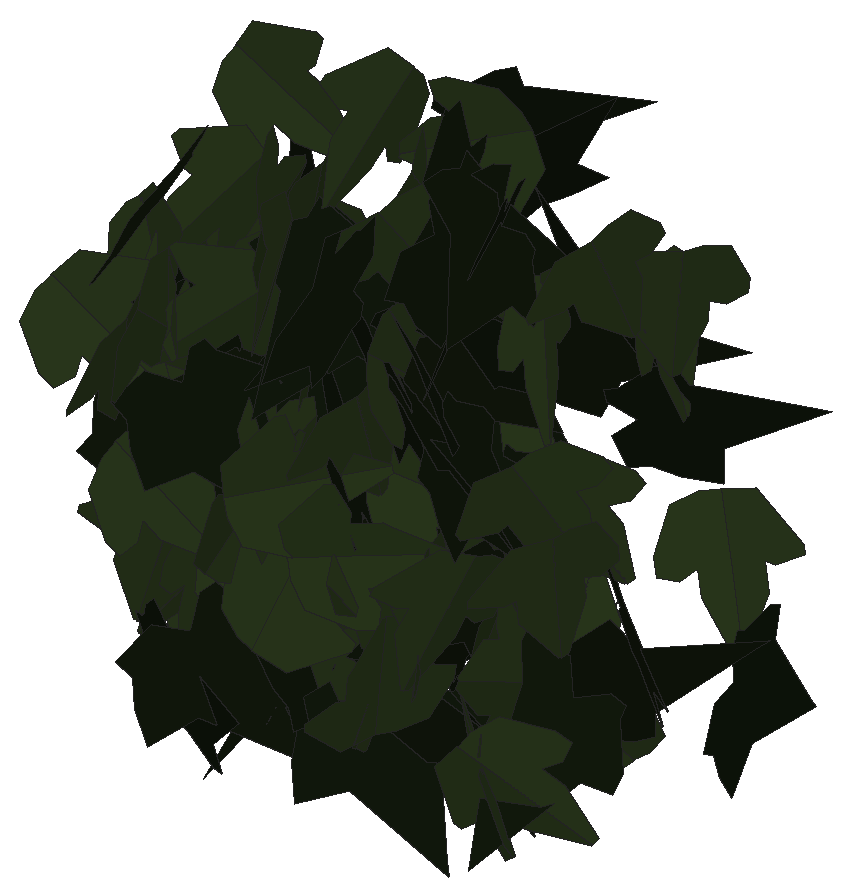
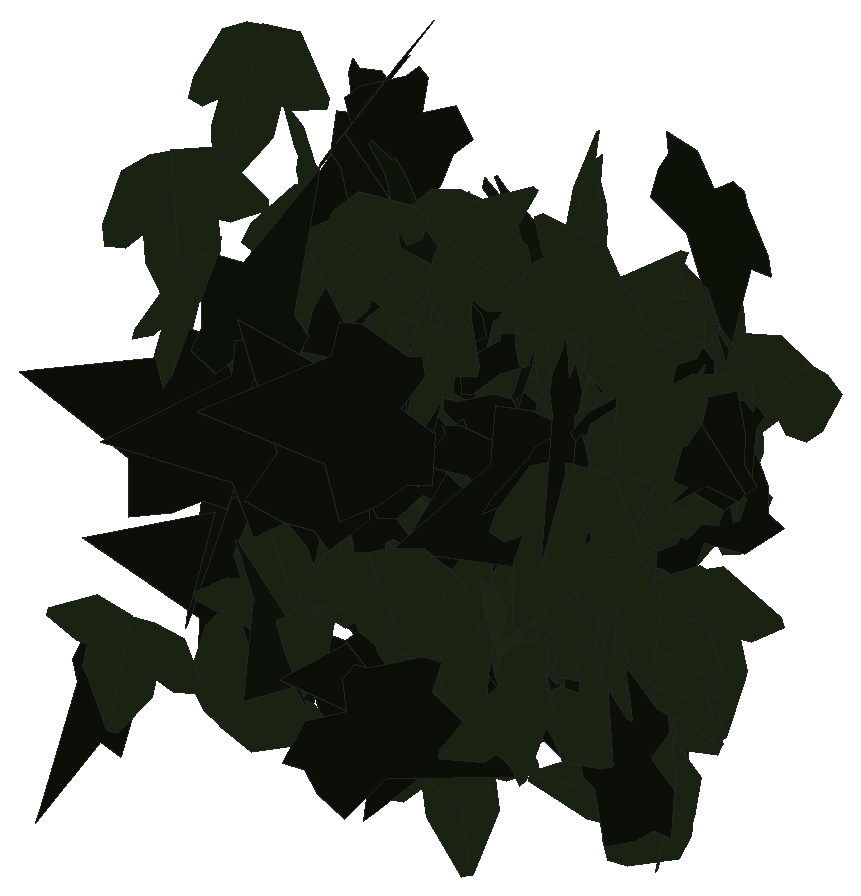
# SketchUp Ruby script. Lengths in inches.
U = 1.inch
M = Sketchup.active_model
def pt(a) = Geom::Point3d.new(a.map { |v| v * U })
def face(e, loops, mat)
  f = e.add_face(loops[0].map { |a| pt(a) })
  loops[1..].each { |l| e.add_face(l.map { |a| pt(a) }).erase! }
  f.material = f.back_material = mat if mat
  f
end
# faces: each face lists its corners as indices into pts; further lists are holes
def faces(e, pts, list, mat = nil) = list.each { |f| face(e, (f[0].is_a?(Array) ? f : [f]).map { |l| l.map { |i| pts[i] } }, mat) }
# xy, xz, yz: faces in a plane at the given z, y or x. An outline is a flat list of corners, or four numbers for a rectangle; further outlines are holes
def ring(l) = l.size == 4 ? [[l[0], l[1]], [l[2], l[1]], [l[2], l[3]], [l[0], l[3]]] : l.each_slice(2).to_a
def flat(e, list, mat, &to3) = list.each { |f| face(e, (f[0].is_a?(Array) ? f : [f]).map { |l| ring(l).map { |u, v| to3.(u, v) } }, mat) }
def xy(e, z, list, mat = nil) = flat(e, list, mat) { |x, y| [x, y, z] }
def xz(e, y, list, mat = nil) = flat(e, list, mat) { |x, z| [x, y, z] }
def yz(e, x, list, mat = nil) = flat(e, list, mat) { |y, z| [x, y, z] }
def lines(e, pts, list) = list.each { |a, b| e.add_line(pt(pts[a]), pt(pts[b])) }
# prism: a flat outline (further loops are holes) pulled along v
def prism(e, loops, v, mat = nil)
  f = face(e, loops, mat); d = Geom::Vector3d.new(v.map { |x| x * U })
  f.pushpull(f.normal.samedirection?(d) ? d.length : -d.length)
end
def box(e, o, s, mat = nil) = prism(e, [[o, [o[0] + s[0], o[1], o[2]], [o[0] + s[0], o[1] + s[1], o[2]], [o[0], o[1] + s[1], o[2]]]], [0, 0, s[2]], mat)
def at(x, y, z, deg = 0) = Geom::Transformation.translation(pt([x, y, z])) * Geom::Transformation.rotation(ORIGIN, Z_AXIS, deg.degrees)
def axes(o, x, y, z) = Geom::Transformation.new([*x, 0, *y, 0, *z, 0, *pt(o).to_a, 1])
def part(name) = M.definitions.add(name)
# library, detail: a bought-in or finely detailed component or shape, given as its bounding box
def library(name, o, s) = part(name).tap { |d| box(d.entities, o, s) }
def detail(e, o, s) = box(e.add_group.entities, o, s)
def put(e, d, t, mat = nil) = e.add_instance(d, t).tap { |i| i.material = mat if mat }
def group(e, t, mat = nil) = e.add_group.tap { |g| g.transformation = t; g.material = mat if mat }.entities
root = M.entities
M.materials.add("efeu1").color = [18, 25, 13]
M.materials.add("efeu2").color = [43, 57, 29]
c1 = part("ivyleaf_10")
p = [[0,0.5,-0.03],[-0.0625,2.02,-0.43],[-0.19,2.01,-0.46],[-0.54,1.05,-0.29],[-0.52,0.625,-0.18],[-0.83,0.76,-0.28],
  [-1.16,0.64,-0.33],[-1.15,0.33,-0.24],[-0.77,-0.39,0.02],[-0.3,-0.51,0.16],[0.04,-0.48,0.23],[-0.02,2.01,-0.4375],
  [-0.06,2.01,-0.43],[0.04,-0.49,0.23],[0.67,-0.49,0.14],[1.38,0.36,-0.2],[1.375,0.51,-0.24],[0.81,0.65,-0.19],
  [0.62,0.59,-0.15],[0.6,1.09,-0.28],[0.5,1.23,-0.31]]
faces(c1.entities,p,[[0,1,2,3,4,5,6,7,8,9,10],[11,12,0,13,14,15,16,17,18,19,20]],"efeu2")
c2 = part("ivyleaf_9")
p = [[1.54,2.16,1.25],[1.36,2.04,1.19],[-0.21,0.99,0.68],[-0.71,1.11,0.82],[-0.85,0.86,0.67],[-0.8,0.17,0.21],
  [-0.9,-0.01,0.1],[-0.67,-0.16,-0.02],[-0.08,-0.08,-0.05],[-0.03,-0.6,-0.4],[0.65,-0.88,-0.66],[0.83,-0.6,-0.49],
  [1.29,-0.42,-0.43],[1.8125,-0.07,-0.26],[1.21,0.44,0.15]]
faces(c2.entities,p,[[0,1,2,3,4,5,6,7,8,9,10,11,12,13,14]],"efeu1")
put(root,c1,axes([28.36,223.71,203.66],[0.46566,0.01688,-0.18132],[0.18117,0.00738,0.46597],[0.0184,-0.49966,0.00076]))
put(root,c1,axes([29.96,224.01,204.44],[-0.14078,-0.43807,0.19564],[-0.05669,-0.18727,-0.46013],[0.47641,-0.15174,0.00306]))
put(root,c1,axes([28.4,223.55,204.82],[-0.03359,-0.06371,0.49479],[0.20668,0.44957,0.07192],[-0.45404,0.20936,-0.00387]))
put(root,c1,axes([28.33,224.03,204.2],[-0.08027,0.02362,-0.49295],[0.40117,-0.28775,-0.07911],[-0.28743,-0.40822,0.02725]))
put(root,c1,axes([30.4375,223.75,203.14],[-0.3156,-0.0886,-0.37755],[0.36635,0.09157,-0.32772],[0.12722,-0.48349,0.00712]))
put(root,c1,axes([30.99,223.85,205.05],[-0.22617,-0.44065,-0.06837],[0.03381,0.05949,-0.4953],[0.44464,-0.22866,0.00288]))
put(root,c1,axes([29.2,224.02,203],[-0.20347,-0.45235,-0.0631],[-0.00825,-0.06542,0.49563],[-0.45665,0.20273,0.01916]))
put(root,c1,axes([28,223.69,204.17],[0.04289,-0.36939,0.33423],[-0.05554,0.32983,0.37165],[-0.49505,-0.06901,-0.01274]))
put(root,c1,axes([30.53,223.76,202.63],[-0.27978,0.29636,-0.28965],[-0.20413,0.20558,0.40751],[0.36063,0.34628,0.00596]))
put(root,c2,axes([27.23,223.64,206.8],[-0.10665,0.44879,0.19291],[-0.04696,0.18712,-0.46128],[-0.48623,-0.1165,0.00224]))
put(root,c1,axes([30.31,224.23,203.57],[-0.12373,0.22145,0.43087],[0.18217,-0.3908,0.25317],[0.4489,0.21963,0.01602]))
put(root,c1,axes([28.82,223.75,204.31],[-0.08375,-0.06088,0.48916],[0.37642,0.31246,0.10334],[-0.31826,0.38557,-0.00651]))
put(root,c1,axes([28.01,224.26,206.53],[0.08941,-0.14177,0.47107],[0.30496,-0.35971,-0.16614],[0.38601,0.31703,0.02215]))
put(root,c2,axes([27.61,223.76,203.23],[0.01041,-0.22486,-0.44647],[0.01909,0.44642,-0.22438],[0.49953,-0.01238,0.01788]))
put(root,c2,axes([27.07,224.18,202.4375],[0.08201,-0.12595,0.47688],[0.25522,-0.40284,-0.15029],[0.42206,0.26807,-0.00179]))
put(root,c1,axes([26.78,223.91,205.47],[0.04597,-0.476,-0.146],[-0.00258,0.14639,-0.47808],[0.49788,0.0447,0.011]))
put(root,c2,axes([27.43,223.89,205.24],[-0.06272,-0.14587,-0.47412],[0.30333,0.36686,-0.153],[0.3925,-0.30682,0.04247]))
put(root,c1,axes([27.1,223.78,205.84],[0.01957,-0.32893,-0.37606],[0.02984,0.37644,-0.32772],[0.49872,-0.00962,0.03437]))
put(root,c1,axes([26.36,223.86,205.64],[0.24713,0.23543,0.36538],[0.26925,0.24703,-0.34129],[-0.34122,0.36544,-0.00468]))
put(root,c1,axes([30.625,224,205.52],[-0.31439,-0.31233,-0.23153],[0.16387,0.16356,-0.44316],[0.35257,-0.35454,-0.00048]))
put(root,c2,axes([30.73,224.36,203.48],[-0.42963,-0.25175,-0.04522],[0.03834,0.02402,-0.49795],[0.25289,-0.43133,-0.00134]))
put(root,c1,axes([26.95,223.9,204.4],[0.14065,0.37067,0.30466],[0.11794,0.28104,-0.39637],[-0.46509,0.18336,-0.00837]))
put(root,c1,axes([29.35,224.46,204],[0.15839,-0.1638,0.44506],[0.30575,-0.32343,-0.22784],[0.36253,0.34433,-0.0023]))
put(root,c2,axes([28.74,224.1875,206.4],[-0.41919,0.27118,-0.02732],[0.02259,-0.01537,-0.49925],[-0.27161,-0.41979,0.00063]))
put(root,c1,axes([28.92,224.1,205.48],[-0.13501,-0.45118,-0.16796],[0.03913,0.16358,-0.47086],[0.47984,-0.14028,-0.00886]))
put(root,c1,axes([28.27,224.2,203.11],[-0.38203,-0.14243,0.28942],[0.27076,0.10227,0.40772],[-0.17534,0.46825,-0.00101]))
put(root,c2,axes([29.36,224.2,205.67],[0.42518,-0.25677,-0.05739],[-0.04797,0.03158,-0.49669],[0.25869,0.42787,0.00222]))
put(root,c1,axes([26.6,224.375,206.13],[0.34341,-0.09658,0.35034],[0.34305,-0.07293,-0.35637],[0.11994,0.48513,0.01618]))
put(root,c1,axes([27.6,224.47,205.89],[-0.20004,-0.23101,0.39575],[-0.26277,-0.29594,-0.30557],[0.37541,-0.33024,-0.00301]))
put(root,c1,axes([29.11,224.2,203.99],[-0.35797,-0.33262,-0.10594],[0.07823,0.07145,-0.48865],[0.3402,-0.36641,0.00089]))
put(root,c1,axes([26.91,224.33,203.69],[-0.41867,-0.22008,0.16211],[-0.14267,-0.077,-0.47299],[0.23316,-0.44231,0.00168]))
put(root,c2,axes([29.75,224.74,207.07],[-0.04366,-0.37256,0.3306],[0.0047,-0.33216,-0.37369],[0.49807,-0.02953,0.03251]))
put(root,c2,axes([29.06,224.21,205.875],[0.30943,-0.00816,-0.39266],[-0.39265,0.00451,-0.30952],[0.0086,0.49991,-0.00362]))
put(root,c2,axes([26.91,224.21,204.25],[-0.21816,0.00004,0.4499],[0.4498,0.01043,0.21811],[-0.00937,0.49989,-0.00459]))
put(root,c1,axes([28.06,224,204.77],[0.07839,0.01655,-0.49354],[0.03315,0.49842,0.02198],[0.4927,-0.03616,0.07705]))
put(root,c2,axes([29.69,224.25,205.37],[0.29056,-0.23019,-0.33554],[-0.22717,0.2503,-0.36843],[0.33759,0.36655,0.04087]))
put(root,c1,axes([26.71,224.43,204.96],[-0.07881,-0.00041,0.49375],[0.48655,0.08504,0.07773],[-0.08404,0.49271,-0.01301]))
put(root,c2,axes([28.7,224.37,204.51],[0.03214,-0.33618,0.36872],[-0.0266,0.3678,0.33766],[-0.49826,-0.04132,0.00576]))
put(root,c2,axes([29.08,224.77,205.56],[0.06667,-0.25591,0.42434],[0.15952,-0.39429,-0.26285],[0.46916,0.17043,0.02907]))
put(root,c2,axes([28.35,224.43,202.875],[-0.09901,-0.39466,0.29058],[0.11898,0.26823,0.40484],[-0.47544,0.14931,0.0408]))
put(root,c2,axes([28.72,224.45,202.71],[-0.02289,-0.3569,-0.34942],[0.03377,0.34788,-0.35754],[0.49833,-0.03997,0.00818]))
put(root,c1,axes([27.13,224.63,203.46],[0.11666,0.43581,-0.21555],[-0.05447,-0.20856,-0.45115],[-0.48314,0.12874,-0.00119]))
put(root,c1,axes([29.15,224.17,205.95],[-0.09196,0.28444,0.4008],[-0.16004,0.3682,-0.29802],[-0.46468,-0.1831,0.02333]))
put(root,c1,axes([28.86,224.36,202.7],[0.18512,-0.38408,0.26117],[-0.11654,0.23374,0.42636],[-0.44961,-0.21873,-0.00298]))
put(root,c2,axes([26.66,224.67,205],[-0.13663,-0.04022,0.47929],[0.40601,-0.27676,0.09252],[0.25786,0.41447,0.10828]))
put(root,c2,axes([28.65,224.38,202.76],[0.08128,0.09539,-0.48404],[0.26104,0.40795,0.12423],[0.41863,-0.2729,0.01651]))
put(root,c1,axes([27.4,224.49,203.27],[0.34875,0.07642,-0.35005],[0.34289,0.07051,0.35701],[0.10393,-0.48907,-0.00323]))
put(root,c2,axes([29.72,224.79,207.09],[-0.27056,0.19985,-0.36994],[0.28929,-0.23077,-0.33624],[-0.30514,-0.39599,0.00925]))
put(root,c1,axes([26.65,224.9,205.01],[-0.09092,-0.38897,-0.30073],[-0.07898,-0.2903,0.39936],[-0.48528,0.12012,-0.00866]))
put(root,c1,axes([27.86,224.28,206.73],[0,-0.0654,-0.4957],[-0.07457,0.49016,-0.06467],[0.49441,0.07393,-0.00975]))
put(root,c2,axes([27.85,224.68,202.79],[-0.37127,0.29932,-0.1502],[0.11677,-0.09448,-0.47691],[-0.31388,-0.3892,0.00025]))
put(root,c1,axes([30.07,224.8,206.47],[0.3738,-0.13957,0.30132],[0.2803,-0.11067,-0.39898],[0.17806,0.4672,-0.00449]))
put(root,c1,axes([28.07,224.39,203.7],[-0.04914,-0.25071,0.4298],[0.11392,0.41475,0.25495],[-0.48436,0.12298,0.01636]))
put(root,c1,axes([26.59,224.9375,202.6],[-0.09541,0.22542,-0.43598],[0.12342,-0.41885,-0.24357],[-0.47504,-0.1541,0.02428]))
put(root,c2,axes([28.4,224.4,204.625],[0.08216,-0.0597,-0.48958],[-0.11328,0.48077,-0.07764],[0.48002,0.12367,0.06547]))
put(root,c1,axes([26.97,225.08,206.41],[-0.08411,-0.20791,0.44688],[0.00299,-0.45355,-0.21045],[0.49286,-0.03273,0.07754]))
put(root,c2,axes([28.05,225.1,205.92],[-0.18681,-0.41009,0.21663],[-0.09088,-0.19665,-0.45063],[0.4548,-0.20774,-0.00107]))
put(root,c1,axes([26.97,225.02,203.34],[-0.08653,-0.32308,0.37166],[-0.09141,-0.36026,-0.33445],[0.4839,-0.12583,0.00328]))
put(root,c1,axes([26.8,225.09,203.81],[-0.02162,-0.31712,0.38597],[-0.01491,-0.38574,-0.31777],[0.49931,-0.02525,0.00722]))
put(root,c2,axes([26.625,224.5,205.61],[0.41705,0.26964,0.05801],[0.04821,0.03228,-0.49662],[-0.27156,0.41982,0.00092]))
put(root,c2,axes([28.5,224.88,204.81],[-0.21636,-0.15295,-0.42402],[-0.34569,-0.24555,0.26496],[-0.28929,0.40781,0.00051]))
put(root,c2,axes([29.44,224.43,207.03],[0.08854,0.00695,-0.49205],[-0.14415,0.47839,-0.01918],[0.47051,0.14525,0.08672]))
put(root,c1,axes([26.71,225.16,205.65],[-0.01071,0.00375,-0.49987],[-0.19466,-0.46055,0.00072],[-0.46043,0.19462,0.01132]))
put(root,c1,axes([26.92,225.21,205.58],[-0.01961,-0.08562,0.49223],[0.10652,-0.482,-0.07959],[0.48813,0.10174,0.03714]))
put(root,c1,axes([30.74,224.71,207.2],[-0.17851,-0.42333,-0.1973],[0.07735,0.18151,-0.45943],[0.4606,-0.19454,0.00069]))
put(root,c1,axes([27.97,225.07,203.41],[0.10914,-0.44559,0.19884],[0.04328,-0.19411,-0.45875],[0.48602,0.11735,-0.0038]))
put(root,c1,axes([28.86,224.73,204.58],[0.10314,0.08368,0.48204],[0.37603,0.3016,-0.13282],[-0.31299,0.38992,-0.00072]))
put(root,c1,axes([30.22,224.86,204.91],[-0.34798,-0.25992,-0.24769],[0.21333,0.12776,-0.43378],[0.28879,-0.40758,0.02198]))
put(root,c2,axes([29.25,225.2,202.22],[0.14758,-0.17942,0.44275],[0.25884,-0.35945,-0.23194],[0.40153,0.29766,-0.01321]))
put(root,c2,axes([29.17,225.07,203.21],[-0.25966,-0.02031,0.42681],[0.37252,-0.2554,0.21448],[0.2093,0.42937,0.14776]))
put(root,c1,axes([27.25,225.18,204.87],[-0.28575,-0.32377,0.25204],[-0.16894,-0.18705,-0.43182],[0.3739,-0.33195,-0.0025]))
put(root,c1,axes([29.53,224.98,203.35],[0.13343,-0.46045,0.14205],[-0.04029,0.13622,0.4794],[-0.48018,-0.13938,-0.00075]))
put(root,c1,axes([28.59,224.9375,206.6],[-0.28679,-0.31882,-0.25711],[0.16771,0.19495,-0.4288],[0.37367,-0.33219,-0.00489]))
put(root,c1,axes([27.36,225.05,205.88],[-0.3069,0.38985,-0.06186],[0.03841,-0.0485,-0.49616],[-0.39286,-0.3093,-0.00018]))
put(root,c2,axes([29.16,224.99,205.9],[0.27835,0.25887,-0.32482],[-0.24971,-0.20817,-0.37988],[-0.33191,0.3737,0.0134]))
put(root,c1,axes([28.59,225.11,202.3],[-0.44313,-0.1929,0.12814],[-0.11734,-0.0515,-0.4833],[0.19966,-0.45841,0.00037]))
put(root,c2,axes([30.8125,224.92,204.05],[0.31443,-0.05255,-0.38519],[-0.37126,0.10637,-0.31757],[0.11532,0.48572,0.02787]))
put(root,c1,axes([27.9375,225.33,203.98],[0.1959,-0.40032,0.22665],[0.10168,-0.20258,-0.44567],[0.44865,0.2207,0.00204]))
put(root,c1,axes([27.88,225.0625,204.71],[0.39459,0.20538,0.2283],[0.20326,0.10397,-0.44484],[-0.23019,0.44386,-0.00144]))
put(root,c1,axes([26.9,225.23,203.05],[-0.19982,-0.45748,-0.02802],[-0.01105,-0.02575,0.49921],[-0.4582,0.20013,0.00017]))
put(root,c2,axes([28.9,225.04,204.32],[-0.35915,-0.08725,0.33674],[0.33877,0.02221,0.36707],[-0.07901,0.49183,0.04316]))
put(root,c2,axes([27.88,225.38,205.1875],[-0.37973,-0.28368,-0.15917],[0.12541,0.09807,-0.47398],[0.30013,-0.39989,-0.00333]))
put(root,c1,axes([27.59,225.21,206.5],[0.05454,-0.4933,-0.06065],[-0.00667,0.06028,-0.49631],[0.49697,0.05494,-0.00001]))
put(root,c2,axes([29.13,224.97,205.82],[0.16893,-0.17258,-0.43781],[-0.20726,0.39033,-0.23384],[0.4225,0.26049,0.06034]))
put(root,c1,axes([26.87,225.19,204.25],[-0.43039,0.12597,-0.22112],[0.21446,-0.05435,-0.44839],[-0.137,-0.48081,-0.00725]))
put(root,c1,axes([27.78,224.86,205.08],[0.03118,-0.01227,-0.49888],[-0.07674,0.49379,-0.01695],[0.49309,0.07762,0.02891]))
put(root,c1,axes([28.34,225.0625,203.33],[0.34784,0.14379,-0.32914],[0.29819,0.13983,0.37621],[0.20024,-0.45801,0.01152]))
put(root,c1,axes([28.93,225.2,205.17],[-0.09633,-0.469,0.14408],[0.03245,0.14042,0.47878],[-0.48956,0.10159,0.00339]))
put(root,c1,axes([26.5625,225.1,202.45],[-0.04534,-0.08229,0.49109],[0.40899,0.27513,0.08387],[-0.28403,0.40931,0.04236]))
put(root,c1,axes([29.63,225.28,203.46],[-0.32375,0.37871,0.042],[0.01388,-0.04335,0.49792],[0.38078,0.32358,0.01756]))
put(root,c1,axes([27.28,225.19,205.13],[-0.35077,-0.01988,-0.35576],[0.35523,0.01949,-0.35133],[0.02784,-0.49922,0.00045]))
put(root,c1,axes([27.06,225.125,205.14],[-0.14167,-0.17356,-0.447],[0.41923,0.18141,-0.20331],[0.23275,-0.4324,0.09412]))
put(root,c2,axes([30.34,225.05,203.07],[0.16779,0.01888,0.47063],[0.43774,0.17819,-0.16321],[-0.17388,0.46679,0.04327]))
put(root,c2,axes([26.52,225.35,203.01],[0.22302,-0.01698,-0.44718],[0.4115,0.20415,0.19747],[0.17588,-0.45611,0.10504]))
put(root,c1,axes([29.98,225.23,203.05],[0.42993,0.22719,-0.1164],[0.1002,0.05949,0.48623],[0.23478,-0.44141,0.00562]))
put(root,c2,axes([28.92,225.05,206.71],[-0.35508,0.20674,-0.28491],[-0.24666,0.14261,0.41088],[0.25115,0.43234,0.00072]))
put(root,c1,axes([26.68,225.21,205.03],[0.16258,0.43277,0.19047],[0.06072,0.18063,-0.46226],[-0.46891,0.17344,0.00618]))
put(root,c1,axes([27.04,225.0625,205.43],[-0.05225,0.32544,0.37598],[-0.04962,0.37275,-0.32954],[-0.49478,-0.07175,-0.00665]))
put(root,c1,axes([27.36,225.08,204.55],[-0.01868,0.28178,0.41262],[-0.06876,0.40753,-0.28141],[-0.4949,-0.06725,0.02353]))
put(root,c2,axes([28.58,225.08,202.97],[0.17251,0.43481,0.17658],[0.06878,0.16268,-0.46777],[-0.46423,0.18568,-0.00369]))
put(root,c2,axes([28.67,225.1,202.85],[0.15068,0.105,0.46505],[0.31453,0.34463,-0.17972],[-0.35828,0.34671,0.03781]))
put(root,c1,axes([30.12,225.64,202.37],[-0.34784,-0.14291,-0.32952],[-0.30054,-0.13539,0.37596],[-0.19669,0.45961,0.00829]))
put(root,c2,axes([30.1,225.12,202.88],[-0.00092,0.27686,0.41635],[-0.00125,0.41635,-0.27686],[-0.5,-0.00155,-0.00007]))
put(root,c1,axes([27.83,225.86,207.07],[-0.06682,-0.33167,0.36815],[0.0653,-0.37413,-0.32521],[0.49119,0.00462,0.09331]))
put(root,c1,axes([26.75,225.59,207.01],[0.24015,0.06087,0.43431],[0.39675,0.18082,-0.24472],[-0.18686,0.46217,0.03854]))
put(root,c2,axes([27.03,225.73,205.64],[0.14269,-0.42973,-0.21205],[-0.06953,0.20034,-0.4528],[0.47413,0.15871,-0.00259]))
put(root,c1,axes([30.7,225.75,206.59],[-0.3038,-0.39663,0.01982],[-0.00984,-0.01742,-0.4996],[0.397,-0.30394,0.00278]))
put(root,c1,axes([28.17,225.75,203.12],[-0.34003,-0.11848,0.3469],[0.34165,0.06909,0.35848],[-0.13288,0.48082,0.03398]))
put(root,c1,axes([27.85,225.86,202.66],[0.35022,-0.16287,-0.31752],[0.28358,-0.14305,0.38616],[-0.21663,-0.45056,-0.00782]))
put(root,c2,axes([27.02,225.78,205.23],[0.4519,-0.06908,0.20251],[0.19878,-0.03955,-0.45708],[0.07917,0.49362,-0.00828]))
put(root,c2,axes([29.75,226.1,205.71],[0.33371,-0.30838,0.20866],[-0.14723,0.14807,0.45431],[-0.34199,-0.36466,0.00802]))
put(root,c2,axes([26.95,225.74,206.17],[0.0288,0.01523,-0.49894],[-0.44171,0.23358,-0.01836],[0.23252,0.44183,0.02691]))
put(root,c1,axes([28.0625,225.84,206.41],[0.05694,-0.38569,-0.31305],[0.02728,0.31705,-0.38566],[0.496,0.02684,0.05715]))
put(root,c1,axes([28.71,226.07,206.93],[0.22539,0.03257,-0.44513],[-0.44451,0.06115,-0.22061],[0.04007,0.49518,0.05652]))
put(root,c1,axes([27.91,225.68,203.96],[0.04022,0.04984,-0.49588],[0.1054,0.48539,0.05733],[0.48711,-0.10914,0.02854]))
put(root,c1,axes([26.78,225.98,205.39],[-0.23088,-0.3931,-0.20534],[0.10626,0.17572,-0.45588],[0.43058,-0.25415,0.00239]))
put(root,c1,axes([30.26,226.06,206.09],[-0.07645,0.49237,0.04159],[-0.01463,0.03981,-0.4982],[-0.4939,-0.07739,0.00832]))
put(root,c1,axes([28.24,226.36,204.41],[0.44387,0.20835,-0.09782],[-0.08897,-0.04068,-0.49034],[-0.21229,0.4527,0.00096]))
put(root,c2,axes([30.07,226.12,204.93],[0.24693,0.25675,-0.35086],[0.20785,0.28469,0.35461],[0.38187,-0.32099,0.03386]))
put(root,c2,axes([29.2,226.15,205.26],[0.10275,0.23308,-0.43025],[0.16879,0.39577,0.25471],[0.4593,-0.19758,0.00265]))
put(root,c1,axes([27.01,226.125,203.74],[0.00654,-0.07673,-0.49403],[0.12113,0.4796,-0.07289],[0.48506,-0.11873,0.02486]))
put(root,c2,axes([30.78,226.34,202.79],[0.05905,0.00273,-0.49649],[-0.34731,0.35753,-0.03934],[0.35481,0.34952,0.04412]))
put(root,c2,axes([27.83,227.19,203.71],[-0.02763,-0.01075,-0.49912],[-0.04593,-0.49771,0.01327],[-0.49712,0.04658,0.02651]))
put(root,c1,axes([30.02,227.1,203.58],[0.46014,0.12905,0.14704],[0.14091,0.04207,-0.47788],[-0.13571,0.48122,0.00235]))
put(root,c2,axes([27.86,227.07,205.72],[0.31659,0.38672,-0.01488],[0.00917,0.01172,0.49978],[0.38689,-0.31672,0.00032]))
put(root,c2,axes([27.64,226.96,206.28],[0.10044,0.30242,-0.38529],[0.13246,0.36189,0.31858],[0.47156,-0.16607,-0.00742]))
